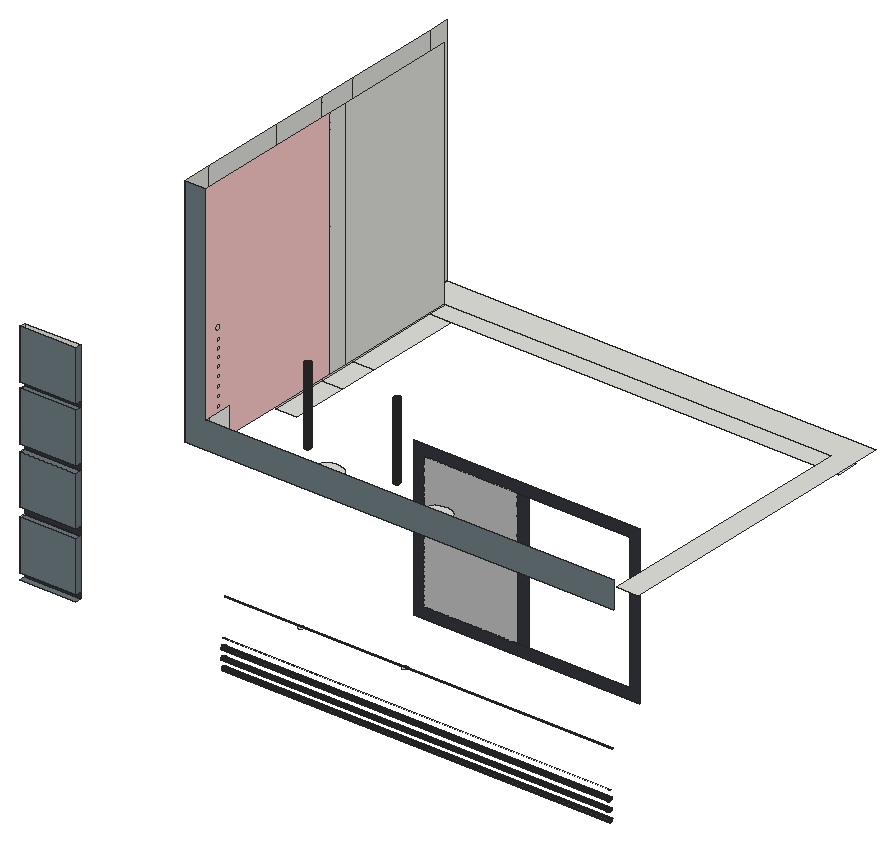
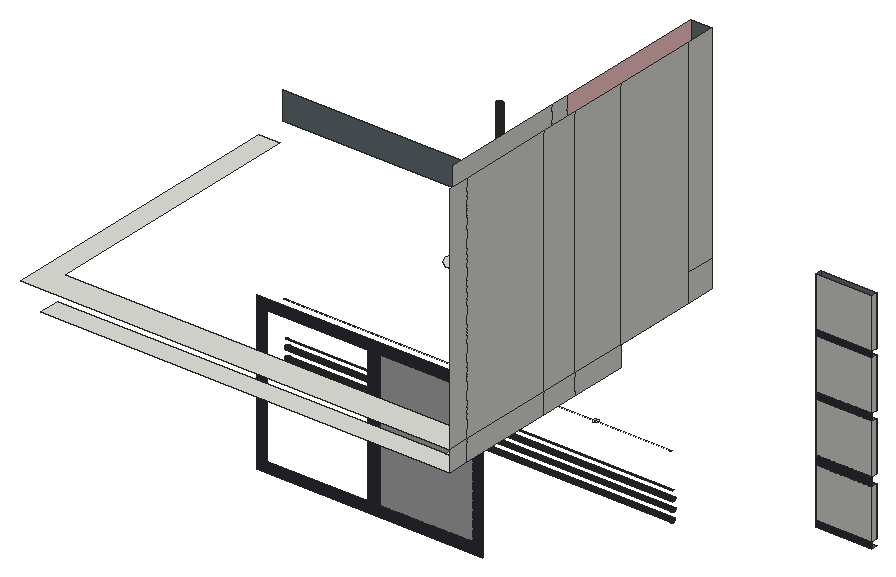
# SketchUp Ruby script. Lengths in inches.
U = 1.inch
M = Sketchup.active_model
def pt(a) = Geom::Point3d.new(a.map { |v| v * U })
def face(e, loops, mat)
  f = e.add_face(loops[0].map { |a| pt(a) })
  loops[1..].each { |l| e.add_face(l.map { |a| pt(a) }).erase! }
  f.material = f.back_material = mat if mat
  f
end
# faces: each face lists its corners as indices into pts; further lists are holes
def faces(e, pts, list, mat = nil) = list.each { |f| face(e, (f[0].is_a?(Array) ? f : [f]).map { |l| l.map { |i| pts[i] } }, mat) }
# xy, xz, yz: faces in a plane at the given z, y or x. An outline is a flat list of corners, or four numbers for a rectangle; further outlines are holes
def ring(l) = l.size == 4 ? [[l[0], l[1]], [l[2], l[1]], [l[2], l[3]], [l[0], l[3]]] : l.each_slice(2).to_a
def flat(e, list, mat, &to3) = list.each { |f| face(e, (f[0].is_a?(Array) ? f : [f]).map { |l| ring(l).map { |u, v| to3.(u, v) } }, mat) }
def xy(e, z, list, mat = nil) = flat(e, list, mat) { |x, y| [x, y, z] }
def xz(e, y, list, mat = nil) = flat(e, list, mat) { |x, z| [x, y, z] }
def yz(e, x, list, mat = nil) = flat(e, list, mat) { |y, z| [x, y, z] }
def lines(e, pts, list) = list.each { |a, b| e.add_line(pt(pts[a]), pt(pts[b])) }
# prism: a flat outline (further loops are holes) pulled along v
def prism(e, loops, v, mat = nil)
  f = face(e, loops, mat); d = Geom::Vector3d.new(v.map { |x| x * U })
  f.pushpull(f.normal.samedirection?(d) ? d.length : -d.length)
end
def box(e, o, s, mat = nil) = prism(e, [[o, [o[0] + s[0], o[1], o[2]], [o[0] + s[0], o[1] + s[1], o[2]], [o[0], o[1] + s[1], o[2]]]], [0, 0, s[2]], mat)
def at(x, y, z, deg = 0) = Geom::Transformation.translation(pt([x, y, z])) * Geom::Transformation.rotation(ORIGIN, Z_AXIS, deg.degrees)
def axes(o, x, y, z) = Geom::Transformation.new([*x, 0, *y, 0, *z, 0, *pt(o).to_a, 1])
def part(name) = M.definitions.add(name)
# library, detail: a bought-in or finely detailed component or shape, given as its bounding box
def library(name, o, s) = part(name).tap { |d| box(d.entities, o, s) }
def detail(e, o, s) = box(e.add_group.entities, o, s)
def put(e, d, t, mat = nil) = e.add_instance(d, t).tap { |i| i.material = mat if mat }
def group(e, t, mat = nil) = e.add_group.tap { |g| g.transformation = t; g.material = mat if mat }.entities
root = M.entities
M.materials.add("[Color A01]").color = [255, 204, 204]
M.materials.add("[Color M06]").color = [86, 86, 86]
M.materials.add("[Formica Laminate Dark]").color = [50, 53, 60]
M.materials.add("[Formica Speckled Grey]").color = [107, 120, 127]
M.materials.add("[Mirror 01]").color = [185, 185, 185]
xy(root,146.25,[[22.92,75.48,40.57,77.29]],"[Formica Speckled Grey]")
xy(root,148.25,[[22.92,75.48,40.57,77.29]],"[Formica Speckled Grey]")
xy(root,157.3125,[[104.45,84,104.64,84.02,104.82,84.1,104.98,84.22,105.1,84.375,105.17,84.55,105.2,84.75,105.17,84.94,105.1,85.125,104.98,85.28,104.82,85.4,104.64,85.47,104.45,85.5,104.25,85.47,104.07,85.4,103.92,85.28,103.8,85.125,103.72,84.94,103.7,84.75,103.72,84.55,103.8,84.375,103.92,84.22,104.07,84.1,104.25,84.02]])
xy(root,157.38,[[137.32,84,137.52,84.02,137.7,84.1,137.85,84.22,137.97,84.375,138.05,84.55,138.07,84.75,138.05,84.93,136.6,84.93,136.57,84.75,136.6,84.55,136.67,84.375,136.79,84.22,136.95,84.1,137.13,84.02],[136.6,84.93,138.05,84.93,138.05,84.94,137.97,85.125,137.85,85.28,137.7,85.4,137.52,85.47,137.32,85.5,137.13,85.47,136.95,85.4,136.79,85.28,136.67,85.125,136.6,84.94]])
xy(root,164,[[22.92,75.48,40.57,77.29]],"[Formica Speckled Grey]")
xy(root,166.81,[[22.92,75.48,40.57,77.29]],"[Formica Speckled Grey]")
xy(root,182.5625,[[22.92,75.48,40.57,77.29]],"[Formica Speckled Grey]")
xy(root,184.81,[[22.92,75.48,40.57,77.29]],"[Formica Speckled Grey]")
xy(root,195.875,[[102.79,91.72,101.62,92.01,100.5625,92.59,99.69,93.43,99.07,94.46,98.73,95.62,98.71,96.83,99,98,99.59,99.06,100.42,99.93,101.46,100.55,102.62,100.89,103.82,100.91,105,100.62,106.05,100.04,106.92,99.2,107.55,98.16,107.88,97,107.9,95.8,107.61,94.625,107.03,93.57,106.19,92.7,105.16,92.07,104,91.74],[137.04,91.72,135.87,92.01,134.8125,92.59,133.94,93.43,133.32,94.46,132.98,95.62,132.96,96.83,133.25,98,133.84,99.06,134.67,99.93,135.71,100.55,136.87,100.89,138.07,100.91,139.25,100.62,140.3,100.04,141.17,99.2,141.8,98.16,142.13,97,142.15,95.8,141.86,94.625,141.28,93.57,140.44,92.7,139.41,92.07,138.25,91.74],[73.48,113.38,80.125,131.65],[73.48,131.65,80.125,143.96],[73.48,143.96,80.125,174.55],
  [73.48,174.55,202.95,181.19]])
xy(root,200.5625,[[22.92,75.48,40.57,77.29]],"[Formica Speckled Grey]")
xy(root,202.375,[[73.48,86.77,73.48,181.19,209.59,181.19,209.59,86.77,202.95,86.77,202.95,171.71,80.125,171.71,80.125,86.77]])
xy(root,202.43,[[22.92,75.48,40.57,77.29]],"[Formica Speckled Grey]")
xy(root,210.9375,[[108.66,81.17,108.4,81.21,108.16,81.31,107.95,81.46,107.8,81.67,107.7,81.91,107.66,82.17,107.7,82.43,107.8,82.67,107.95,82.88,108.16,83.04,108.4,83.14,108.66,83.17,108.92,83.14,109.16,83.04,109.37,82.88,109.53,82.67,109.625,82.43,109.66,82.17,109.625,81.91,109.53,81.67,109.37,81.46,109.16,81.31,108.92,81.21],[136.97,81.17,136.71,81.21,136.47,81.31,136.27,81.46,136.11,81.67,136.01,81.91,135.97,82.17,136.01,82.43,136.11,82.67,136.27,82.88,136.47,83.04,136.71,83.14,136.97,83.17,137.23,83.14,137.47,83.04,137.68,82.88,137.84,82.67,137.9375,82.43,137.97,82.17,137.9375,81.91,137.84,81.67,137.68,81.46,137.47,81.31,137.23,81.21]])
xz(root,75.48,[[22.92,148.25,40.57,164],[22.92,166.81,40.57,182.5625],[22.92,184.81,40.57,200.5625],[22.92,202.43,40.57,218.1875]],"[Formica Speckled Grey]")
xz(root,77.29,[[22.92,148.25,40.57,164],[22.92,166.81,40.57,182.5625],[22.92,184.81,40.57,200.5625],[22.92,202.43,40.57,218.1875]])
xz(root,77.29,[[22.92,146.25,40.57,148.25],[22.92,164,40.57,166.81],[22.92,182.5625,40.57,184.81],[22.92,200.5625,40.57,202.43]],"[Formica Laminate Dark]")
xz(root,77.29,[[73.48,202.375,209.59,202.375,209.59,210.9375,80.125,210.9375,80.125,276.375,73.48,276.375]],"[Formica Speckled Grey]")
xz(root,86.77,[[73.48,202.375,80.125,210.9375]])
xz(root,131.65,[[[102.7,139.62,174.38,189.18],[105.97,142.9,171.11,185.91]],[135.2,142.9,139.18,185.91]],"[Formica Laminate Dark]")
xz(root,131.65,[[105.97,142.9,135.2,185.91]],"[Mirror 01]")
yz(root,22.92,[[75.48,148.25,77.29,164],[75.48,166.81,77.29,182.5625],[75.48,184.81,77.29,200.5625],[75.48,202.43,77.29,218.1875]])
yz(root,40.57,[[75.48,148.25,77.29,164],[75.48,166.81,77.29,182.5625],[75.48,184.81,77.29,200.5625],[75.48,202.43,77.29,218.1875]],"[Formica Speckled Grey]")
yz(root,73.48,[[113.38,195.875,131.65,202.375],[131.65,195.875,143.96,202.375],[143.96,195.875,174.55,202.375],[174.55,195.875,181.19,202.375],[77.29,202.375,86.77,210.9375],
  [86.77,202.375,113.38,276.375],[113.38,202.375,131.65,276.375],[131.65,202.375,143.96,276.375],[143.96,202.375,174.55,276.375],[174.55,202.375,181.19,276.375],
  [77.29,210.9375,86.77,276.375]])
yz(root,80.125,[[126.48,202.375,132.38,276.375],[132.38,202.375,171.71,276.375]])
yz(root,80.125,[[[86.77,202.375,126.48,202.375,126.48,276.375,77.29,276.375,77.29,210.9375,86.77,210.9375],[82.17,234.08,81.91,234.11,81.67,234.21,81.46,234.37,81.3,234.58,81.2,234.82,81.17,235.08,81.2,235.34,81.3,235.58,81.46,235.79,81.67,235.94,81.91,236.04,82.17,236.08,82.42,236.04,82.67,235.94,82.875,235.79,83.03,235.58,83.13,235.34,83.17,235.08,83.13,234.82,83.03,234.58,82.875,234.37,82.67,234.21,82.42,234.11],[82.38,211.9,82.22,211.92,82.07,211.98,81.94,212.08,81.84,212.21,81.78,212.36,81.76,212.52,81.78,212.68,81.84,212.83,81.94,212.96,82.07,213.0625,82.22,213.125,82.38,213.15,82.55,213.125,82.7,213.0625,82.83,212.96,82.92,212.83,82.99,212.68,83.01,212.52,82.99,212.36,82.92,212.21,82.83,212.08,82.7,211.98,82.55,211.92],[82.38,214.83,82.22,214.86,82.07,214.92,81.94,215.02,81.84,215.15,81.78,215.3,81.76,215.46,81.78,215.62,81.84,215.77,81.94,215.9,82.07,216,82.22,216.0625,82.38,216.08,82.55,216.0625,82.7,216,82.83,215.9,82.92,215.77,82.99,215.62,83.01,215.46,82.99,215.3,82.92,215.15,82.83,215.02,82.7,214.92,82.55,214.86],[82.38,217.52,82.22,217.54,82.07,217.61,81.94,217.71,81.84,217.83,81.78,217.99,81.76,218.15,81.78,218.31,81.84,218.46,81.94,218.59,82.07,218.6875,82.22,218.75,82.38,218.77,82.55,218.75,82.7,218.6875,82.83,218.59,82.92,218.46,82.99,218.31,83.01,218.15,82.99,217.99,82.92,217.83,82.83,217.71,82.7,217.61,82.55,217.54],[82.38,220.46,82.22,220.48,82.07,220.54,81.94,220.64,81.84,220.77,81.78,220.92,81.76,221.08,81.78,221.25,81.84,221.4,81.94,221.53,82.07,221.625,82.22,221.6875,82.38,221.71,82.55,221.6875,82.7,221.625,82.83,221.53,82.92,221.4,82.99,221.25,83.01,221.08,82.99,220.92,82.92,220.77,82.83,220.64,82.7,220.54,82.55,220.48],[82.38,223.27,82.22,223.29,82.07,223.36,81.94,223.46,81.84,223.58,81.78,223.74,81.76,223.9,81.78,224.06,81.84,224.21,81.94,224.34,82.07,224.4375,82.22,224.5,82.38,224.52,82.55,224.5,82.7,224.4375,82.83,224.34,82.92,224.21,82.99,224.06,83.01,223.9,82.99,223.74,82.92,223.58,82.83,223.46,82.7,223.36,82.55,223.29],[82.38,225.9,82.22,225.92,82.07,225.98,81.94,226.08,81.84,226.21,81.78,226.36,81.76,226.52,81.78,226.68,81.84,226.83,81.94,226.96,82.07,227.0625,82.22,227.125,82.38,227.15,82.55,227.125,82.7,227.0625,82.83,226.96,82.92,226.83,82.99,226.68,83.01,226.52,82.99,226.36,82.92,226.21,82.83,226.08,82.7,225.98,82.55,225.92],[82.38,228.4,82.22,228.42,82.07,228.48,81.94,228.58,81.84,228.71,81.78,228.86,81.76,229.02,81.78,229.18,81.84,229.33,81.94,229.46,82.07,229.5625,82.22,229.625,82.38,229.65,82.55,229.625,82.7,229.5625,82.83,229.46,82.92,229.33,82.99,229.18,83.01,229.02,82.99,228.86,82.92,228.71,82.83,228.58,82.7,228.48,82.55,228.42],[82.38,230.9,82.22,230.92,82.07,230.98,81.94,231.08,81.84,231.21,81.78,231.36,81.76,231.52,81.78,231.68,81.84,231.83,81.94,231.96,82.07,232.0625,82.22,232.125,82.38,232.15,82.55,232.125,82.7,232.0625,82.83,231.96,82.92,231.83,82.99,231.68,83.01,231.52,82.99,231.36,82.92,231.21,82.83,231.08,82.7,230.98,82.55,230.92]]],"[Color A01]")
p = [[202.95,84,136.84],[202.95,83.87,136.94],[80.125,83.87,136.94],[80.125,84,136.84],[202.95,84.15,136.78],[80.125,84.15,136.78],
  [202.95,84.31,136.76],[80.125,84.31,136.76],[202.95,84.47,136.78],[80.125,84.47,136.78],[202.95,84.62,136.84],[80.125,84.62,136.84],
  [202.95,84.75,136.94],[80.125,84.75,136.94],[202.95,83.77,137.07],[80.125,83.77,137.07],[202.95,84.85,137.07],[80.125,84.85,137.07],
  [202.95,83.7,137.22],[80.125,83.7,137.22],[202.95,84.91,137.22],[80.125,84.91,137.22],[202.95,83.68,137.39],[80.125,83.68,137.39],
  [202.95,84.93,137.39],[80.125,84.93,137.39],[202.95,83.7,137.55],[80.125,83.7,137.55],[202.95,84.91,137.55],[80.125,84.91,137.55],
  [202.95,83.77,137.7],[80.125,83.77,137.7],[202.95,84.85,137.7],[80.125,84.85,137.7],[202.95,83.87,137.83],[80.125,83.87,137.83],
  [202.95,84.75,137.83],[80.125,84.75,137.83],[202.95,84,137.93],[80.125,84,137.93],[202.95,84.62,137.93],[80.125,84.62,137.93],
  [202.95,84.15,137.99],[80.125,84.15,137.99],[202.95,84.47,137.99],[80.125,84.47,137.99],[202.95,84.31,138.01],[80.125,84.31,138.01],
  [202.95,83.98,139.73],[202.95,83.83,139.79],[80.125,83.83,139.79],[80.125,83.98,139.73],[202.95,84.14,139.71],[80.125,84.14,139.71],
  [202.95,84.3,139.73],[80.125,84.3,139.73],[202.95,84.45,139.79],[80.125,84.45,139.79],[202.95,83.7,139.89],[80.125,83.7,139.89],
  [202.95,84.58,139.89],[80.125,84.58,139.89],[202.95,83.6,140.02],[80.125,83.6,140.02],[202.95,84.68,140.02],[80.125,84.68,140.02],
  [202.95,83.54,140.17],[80.125,83.54,140.17],[202.95,84.74,140.17],[80.125,84.74,140.17],[202.95,83.52,140.33],[80.125,83.52,140.33],
  [202.95,84.77,140.33],[80.125,84.77,140.33],[202.95,83.54,140.49],[80.125,83.54,140.49],[202.95,84.74,140.49],[80.125,84.74,140.49],
  [202.95,83.6,140.64],[80.125,83.6,140.64],[202.95,84.68,140.64],[80.125,84.68,140.64],[202.95,83.7,140.77],[80.125,83.7,140.77],
  [202.95,84.58,140.77],[80.125,84.58,140.77],[202.95,83.83,140.87],[80.125,83.83,140.87],[202.95,84.45,140.87],[80.125,84.45,140.87],
  [202.95,83.98,140.93],[80.125,83.98,140.93],[202.95,84.14,140.96],[80.125,84.14,140.96],[202.95,84.3,140.93],[80.125,84.3,140.93],
  [202.95,83.98,142.79],[202.95,83.83,142.85],[80.125,83.83,142.85],[80.125,83.98,142.79],[202.95,84.14,142.77],[80.125,84.14,142.77],
  [202.95,84.3,142.79],[80.125,84.3,142.79],[202.95,84.45,142.85],[80.125,84.45,142.85],[202.95,83.7,142.95],[80.125,83.7,142.95],
  [202.95,84.58,142.95],[80.125,84.58,142.95],[202.95,83.6,143.08],[80.125,83.6,143.08],[202.95,84.68,143.08],[80.125,84.68,143.08],
  [202.95,83.54,143.23],[80.125,83.54,143.23],[202.95,84.74,143.23],[80.125,84.74,143.23],[202.95,83.52,143.39],[80.125,83.52,143.39],
  [202.95,84.77,143.39],[80.125,84.77,143.39],[202.95,83.54,143.56],[80.125,83.54,143.56],[202.95,84.74,143.56],[80.125,84.74,143.56],
  [202.95,83.6,143.71],[80.125,83.6,143.71],[202.95,84.68,143.71],[80.125,84.68,143.71],[202.95,83.7,143.84],[80.125,83.7,143.84],
  [202.95,84.58,143.84],[80.125,84.58,143.84],[202.95,83.83,143.93],[80.125,83.83,143.93],[202.95,84.45,143.93],[80.125,84.45,143.93],
  [202.95,83.98,144],[80.125,83.98,144],[202.95,84.3,144],[80.125,84.3,144],[202.95,84.14,144.02],[80.125,84.14,144.02],
  [202.95,84.31,145.95],[202.95,84.15,145.97],[80.125,84.15,145.97],[80.125,84.31,145.95],[202.95,84.47,145.97],[80.125,84.47,145.97],
  [202.95,84.93,157.38],[202.95,84.82,157.24],[80.125,84.82,157.24],[80.125,84.93,157.38],[136.6,84.93,157.38],[138.05,84.93,157.38],
  [202.95,85,157.54],[80.125,85,157.54],[108.16,81.31,210.9375],[108.4,81.21,210.9375],[108.4,81.21,235.0625],[108.16,81.31,235.0625],
  [108.66,81.17,210.9375],[108.66,81.17,235.0625],[108.92,81.21,210.9375],[108.92,81.21,235.0625],[109.16,81.31,210.9375],[109.16,81.31,235.0625],
  [136.47,81.31,210.9375],[136.71,81.21,210.9375],[136.71,81.21,235],[136.47,81.31,235],[136.97,81.17,210.9375],[136.97,81.17,235],
  [137.23,81.21,210.9375],[137.23,81.21,235],[137.47,81.31,210.9375],[137.47,81.31,235],[107.95,81.46,210.9375],[107.95,81.46,235.0625],
  [109.37,81.46,210.9375],[109.37,81.46,235.0625],[136.27,81.46,210.9375],[136.27,81.46,235],[137.68,81.46,210.9375],[137.68,81.46,235],
  [107.8,81.67,210.9375],[107.8,81.67,235.0625],[109.53,81.67,210.9375],[109.53,81.67,235.0625],[136.11,81.67,210.9375],[136.11,81.67,235],
  [137.84,81.67,210.9375],[137.84,81.67,235],[107.7,81.91,210.9375],[107.7,81.91,235.0625],[109.625,81.91,210.9375],[109.625,81.91,235.0625],
  [136.01,81.91,210.9375],[136.01,81.91,235],[137.9375,81.91,210.9375],[137.9375,81.91,235],[107.66,82.17,210.9375],[107.66,82.17,235.0625],
  [109.66,82.17,210.9375],[109.66,82.17,235.0625],[135.97,82.17,210.9375],[135.97,82.17,235],[137.97,82.17,210.9375],[137.97,82.17,235],
  [107.7,82.43,210.9375],[107.7,82.43,235.0625],[109.625,82.43,210.9375],[109.625,82.43,235.0625],[136.01,82.43,210.9375],[136.01,82.43,235],
  [137.9375,82.43,210.9375],[137.9375,82.43,235],[107.8,82.67,210.9375],[107.8,82.67,235.0625],[109.53,82.67,210.9375],[109.53,82.67,235.0625],
  [136.11,82.67,210.9375],[136.11,82.67,235],[137.84,82.67,210.9375],[137.84,82.67,235],[107.95,82.88,210.9375],[107.95,82.88,235.0625],
  [109.37,82.88,210.9375],[109.37,82.88,235.0625],[136.27,82.88,210.9375],[136.27,82.88,235],[137.68,82.88,210.9375],[137.68,82.88,235],
  [108.16,83.04,210.9375],[108.16,83.04,235.0625],[109.16,83.04,210.9375],[109.16,83.04,235.0625],[136.47,83.04,210.9375],[136.47,83.04,235],
  [137.47,83.04,210.9375],[137.47,83.04,235],[108.4,83.14,210.9375],[108.4,83.14,235.0625],[108.92,83.14,210.9375],[108.92,83.14,235.0625],
  [136.71,83.14,210.9375],[136.71,83.14,235],[137.23,83.14,210.9375],[137.23,83.14,235],[108.66,83.17,210.9375],[108.66,83.17,235.0625],
  [136.97,83.17,210.9375],[136.97,83.17,235]]
faces(root,p,[[0,1,2,3],[4,0,3,5],[6,4,5,7],[8,6,7,9],[10,8,9,11],[12,10,11,13],[1,14,15,2],[16,12,13,17],
  [14,18,19,15],[20,16,17,21],[18,22,23,19],[24,20,21,25],[22,26,27,23],[28,24,25,29],[26,30,31,27],[32,28,29,33],
  [30,34,35,31],[36,32,33,37],[34,38,39,35],[40,36,37,41],[38,42,43,39],[44,40,41,45],[42,46,47,43],[46,44,45,47],
  [48,49,50,51],[52,48,51,53],[54,52,53,55],[56,54,55,57],[49,58,59,50],[60,56,57,61],[58,62,63,59],[64,60,61,65],
  [62,66,67,63],[68,64,65,69],[66,70,71,67],[72,68,69,73],[70,74,75,71],[76,72,73,77],[74,78,79,75],[80,76,77,81],
  [78,82,83,79],[84,80,81,85],[82,86,87,83],[88,84,85,89],[86,90,91,87],[90,92,93,91],[92,94,95,93],[94,88,89,95],
  [96,97,98,99],[100,96,99,101],[102,100,101,103],[104,102,103,105],[97,106,107,98],[108,104,105,109],[106,110,111,107],[112,108,109,113],
  [110,114,115,111],[116,112,113,117],[114,118,119,115],[120,116,117,121],[118,122,123,119],[124,120,121,125],[122,126,127,123],[128,124,125,129],
  [126,130,131,127],[132,128,129,133],[130,134,135,131],[136,132,133,137],[134,138,139,135],[140,136,137,141],[138,142,143,139],[142,140,141,143],
  [144,145,146,147],[148,144,147,149],[150,151,152,153,154,155],[156,150,155,154,153,157],[158,159,160,161],[159,162,163,160],[162,164,165,163],[164,166,167,165],
  [168,169,170,171],[169,172,173,170],[172,174,175,173],[174,176,177,175],[178,158,161,179],[166,180,181,167],[182,168,171,183],[176,184,185,177],
  [186,178,179,187],[180,188,189,181],[190,182,183,191],[184,192,193,185],[194,186,187,195],[188,196,197,189],[198,190,191,199],[192,200,201,193],
  [202,194,195,203],[196,204,205,197],[206,198,199,207],[200,208,209,201],[210,202,203,211],[204,212,213,205],[214,206,207,215],[208,216,217,209],
  [218,210,211,219],[212,220,221,213],[222,214,215,223],[216,224,225,217],[226,218,219,227],[220,228,229,221],[230,222,223,231],[224,232,233,225],
  [234,226,227,235],[228,236,237,229],[238,230,231,239],[232,240,241,233],[242,234,235,243],[236,244,245,237],[246,238,239,247],[240,248,249,241],
  [250,242,243,251],[244,250,251,245],[252,246,247,253],[248,252,253,249]],"[Color M06]")
